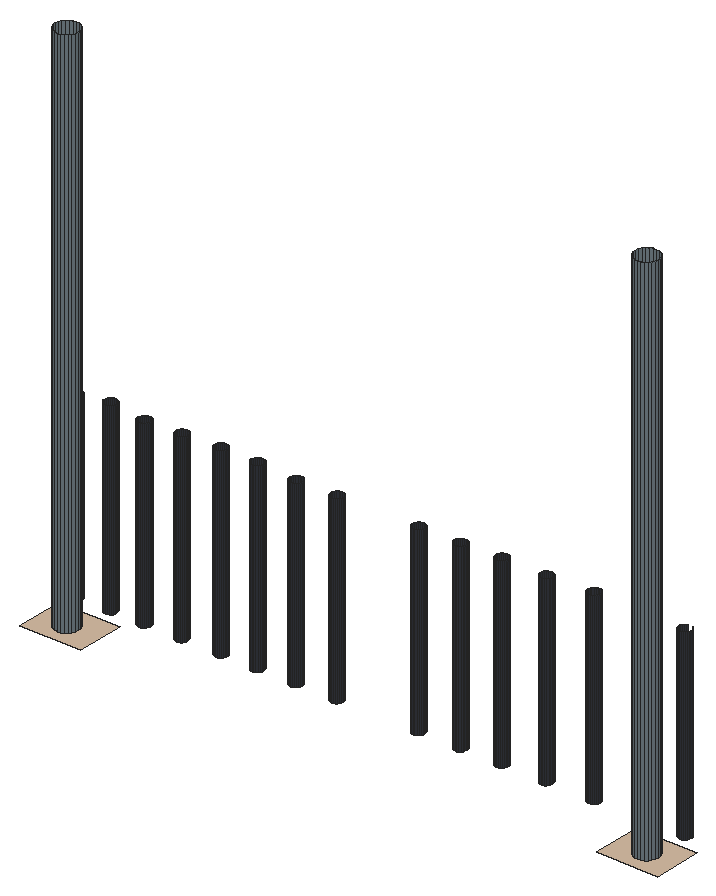
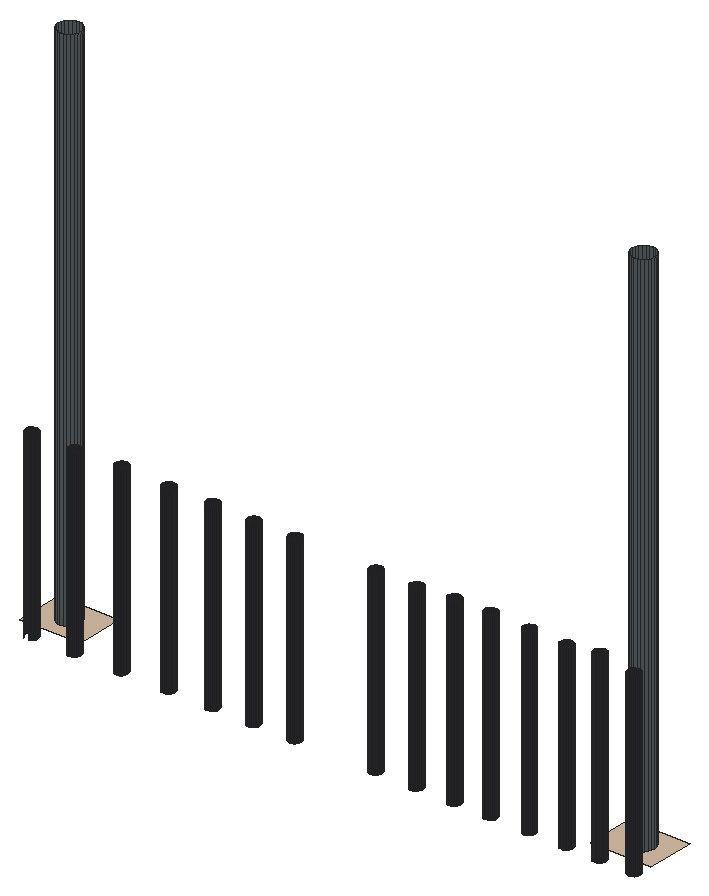
# SketchUp Ruby script. Lengths in inches.
U = 1.inch
M = Sketchup.active_model
def pt(a) = Geom::Point3d.new(a.map { |v| v * U })
def face(e, loops, mat)
  f = e.add_face(loops[0].map { |a| pt(a) })
  loops[1..].each { |l| e.add_face(l.map { |a| pt(a) }).erase! }
  f.material = f.back_material = mat if mat
  f
end
# faces: each face lists its corners as indices into pts; further lists are holes
def faces(e, pts, list, mat = nil) = list.each { |f| face(e, (f[0].is_a?(Array) ? f : [f]).map { |l| l.map { |i| pts[i] } }, mat) }
# xy, xz, yz: faces in a plane at the given z, y or x. An outline is a flat list of corners, or four numbers for a rectangle; further outlines are holes
def ring(l) = l.size == 4 ? [[l[0], l[1]], [l[2], l[1]], [l[2], l[3]], [l[0], l[3]]] : l.each_slice(2).to_a
def flat(e, list, mat, &to3) = list.each { |f| face(e, (f[0].is_a?(Array) ? f : [f]).map { |l| ring(l).map { |u, v| to3.(u, v) } }, mat) }
def xy(e, z, list, mat = nil) = flat(e, list, mat) { |x, y| [x, y, z] }
def xz(e, y, list, mat = nil) = flat(e, list, mat) { |x, z| [x, y, z] }
def yz(e, x, list, mat = nil) = flat(e, list, mat) { |y, z| [x, y, z] }
def lines(e, pts, list) = list.each { |a, b| e.add_line(pt(pts[a]), pt(pts[b])) }
# prism: a flat outline (further loops are holes) pulled along v
def prism(e, loops, v, mat = nil)
  f = face(e, loops, mat); d = Geom::Vector3d.new(v.map { |x| x * U })
  f.pushpull(f.normal.samedirection?(d) ? d.length : -d.length)
end
def box(e, o, s, mat = nil) = prism(e, [[o, [o[0] + s[0], o[1], o[2]], [o[0] + s[0], o[1] + s[1], o[2]], [o[0], o[1] + s[1], o[2]]]], [0, 0, s[2]], mat)
def at(x, y, z, deg = 0) = Geom::Transformation.translation(pt([x, y, z])) * Geom::Transformation.rotation(ORIGIN, Z_AXIS, deg.degrees)
def axes(o, x, y, z) = Geom::Transformation.new([*x, 0, *y, 0, *z, 0, *pt(o).to_a, 1])
def part(name) = M.definitions.add(name)
# library, detail: a bought-in or finely detailed component or shape, given as its bounding box
def library(name, o, s) = part(name).tap { |d| box(d.entities, o, s) }
def detail(e, o, s) = box(e.add_group.entities, o, s)
def put(e, d, t, mat = nil) = e.add_instance(d, t).tap { |i| i.material = mat if mat }
def group(e, t, mat = nil) = e.add_group.tap { |g| g.transformation = t; g.material = mat if mat }.entities
root = M.entities
M.materials.add("[Formica Laminate Dark]").color = [50, 53, 60]
M.materials.add("[Formica Laminate Light]").color = [213, 189, 164]
M.materials.add("[Formica Speckled Grey]").color = [112, 125, 132]
xy(root,372.6,[[299.55,85.05,299.16,85.1,298.8,85.25,298.49,85.49,298.25,85.8,298.1,86.17,298.05,86.55,298.1,86.94,298.25,87.3,298.49,87.61,298.8,87.85,299.16,88,299.55,88.05,299.9375,88,300.3,87.85,300.61,87.61,300.85,87.3,301,86.94,301.05,86.55,301,86.17,300.85,85.8,300.61,85.49,300.3,85.25,299.9375,85.1],[373.86,85.05,373.47,85.1,373.11,85.25,372.8,85.49,372.5625,85.8,372.41,86.17,372.36,86.55,372.41,86.94,372.5625,87.3,372.8,87.61,373.11,87.85,373.47,88,373.86,88.05,374.25,88,374.61,87.85,374.92,87.61,375.16,87.3,375.3125,86.94,375.36,86.55,375.3125,86.17,375.16,85.8,374.92,85.49,374.61,85.25,374.25,85.1]])
xy(root,372.6,[[[295.97,83.54,303.82,89.73],[299.55,85.05,299.16,85.1,298.8,85.25,298.49,85.49,298.25,85.8,298.1,86.17,298.05,86.55,298.1,86.94,298.25,87.3,298.49,87.61,298.8,87.85,299.16,88,299.55,88.05,299.9375,88,300.3,87.85,300.61,87.61,300.85,87.3,301,86.94,301.05,86.55,301,86.17,300.85,85.8,300.61,85.49,300.3,85.25,299.9375,85.1]],[[369.85,83.54,377.7,89.73],[373.86,85.05,373.47,85.1,373.11,85.25,372.8,85.49,372.5625,85.8,372.41,86.17,372.36,86.55,372.41,86.94,372.5625,87.3,372.8,87.61,373.11,87.85,373.47,88,373.86,88.05,374.25,88,374.61,87.85,374.92,87.61,375.16,87.3,375.3125,86.94,375.36,86.55,375.3125,86.17,375.16,85.8,374.92,85.49,374.61,85.25,374.25,85.1]]],"[Formica Laminate Light]")
p = [[298.8,85.25,372.6],[299.16,85.1,372.6],[299.16,85.1,441.22],[298.8,85.25,441.22],[299.55,85.05,372.6],[299.55,85.05,441.22],
  [299.9375,85.1,372.6],[299.9375,85.1,441.22],[300.3,85.25,372.6],[300.3,85.25,441.22],[373.11,85.25,372.6],[373.47,85.1,372.6],
  [373.47,85.1,441.22],[373.11,85.25,441.22],[373.86,85.05,372.6],[373.86,85.05,441.22],[374.25,85.1,372.6],[374.25,85.1,441.22],
  [374.61,85.25,372.6],[374.61,85.25,441.22],[298.49,85.49,372.6],[298.49,85.49,441.22],[300.61,85.49,372.6],[300.61,85.49,441.22],
  [372.8,85.49,372.6],[372.8,85.49,441.22],[374.92,85.49,372.6],[374.92,85.49,441.22],[298.25,85.8,372.6],[298.25,85.8,441.22],
  [300.85,85.8,372.6],[300.85,85.8,441.22],[372.5625,85.8,372.6],[372.5625,85.8,441.22],[375.16,85.8,372.6],[375.16,85.8,441.22],
  [298.1,86.17,372.6],[298.1,86.17,441.22],[301,86.17,372.6],[301,86.17,441.22],[372.41,86.17,372.6],[372.41,86.17,441.22],
  [375.3125,86.17,372.6],[375.3125,86.17,441.22],[298.05,86.55,372.6],[298.05,86.55,441.22],[301.05,86.55,372.6],[301.05,86.55,441.22],
  [372.36,86.55,372.6],[372.36,86.55,441.22],[375.36,86.55,372.6],[375.36,86.55,441.22],[298.1,86.94,372.6],[298.1,86.94,441.22],
  [301,86.94,372.6],[301,86.94,441.22],[372.41,86.94,372.6],[372.41,86.94,441.22],[375.3125,86.94,372.6],[375.3125,86.94,441.22],
  [298.25,87.3,372.6],[298.25,87.3,441.22],[300.85,87.3,372.6],[300.85,87.3,441.22],[372.5625,87.3,372.6],[372.5625,87.3,441.22],
  [375.16,87.3,372.6],[375.16,87.3,441.22],[298.49,87.61,372.6],[298.49,87.61,441.22],[300.61,87.61,372.6],[300.61,87.61,441.22],
  [372.8,87.61,372.6],[372.8,87.61,441.22],[374.92,87.61,372.6],[374.92,87.61,441.22],[298.8,87.85,372.6],[298.8,87.85,441.22],
  [300.3,87.85,372.6],[300.3,87.85,441.22],[373.11,87.85,372.6],[373.11,87.85,441.22],[374.61,87.85,372.6],[374.61,87.85,441.22],
  [299.16,88,372.6],[299.16,88,441.22],[299.9375,88,372.6],[299.9375,88,441.22],[373.47,88,372.6],[373.47,88,441.22],
  [374.25,88,372.6],[374.25,88,441.22],[299.55,88.05,372.6],[299.55,88.05,441.22],[373.86,88.05,372.6],[373.86,88.05,441.22],
  [296.23,90.98,372.6],[296.43,90.9,372.6],[296.43,90.9,395.85],[296.23,90.98,395.85],[296.64,90.87,372.6],[296.64,90.87,395.85],
  [296.85,90.9,372.6],[296.85,90.9,395.85],[297.04,90.98,372.6],[297.04,90.98,395.85],[300.67,90.98,372.6],[300.86,90.9,372.6],
  [300.86,90.9,396.5625],[300.67,90.98,396.5625],[301.07,90.87,372.6],[301.07,90.87,396.5625],[301.28,90.9,372.6],[301.28,90.9,396.5625],
  [301.48,90.98,372.6],[301.48,90.98,396.5625],[304.98,90.98,372.6],[305.18,90.9,372.6],[305.18,90.9,396.04],[304.98,90.98,396.04],
  [305.39,90.87,372.6],[305.39,90.87,396.04],[305.6,90.9,372.6],[305.6,90.9,396.04],[305.79,90.98,372.6],[305.79,90.98,396.04],
  [309.79,90.98,372.6],[309.99,90.9,372.6],[309.99,90.9,396.16],[309.79,90.98,396.16],[310.2,90.87,372.6],[310.2,90.87,396.16],
  [310.41,90.9,372.6],[310.41,90.9,396.16],[310.6,90.98,372.6],[310.6,90.98,396.16],[314.79,90.98,372.6],[314.99,90.9,372.6],
  [314.99,90.9,396.35],[314.79,90.98,396.35],[315.2,90.87,372.6],[315.2,90.87,396.35],[315.41,90.9,372.6],[315.41,90.9,396.35],
  [315.6,90.98,372.6],[315.6,90.98,396.35],[319.48,90.98,372.6],[319.68,90.9,372.6],[319.68,90.9,396.29],[319.48,90.98,396.29],
  [319.89,90.87,372.6],[319.89,90.87,396.29],[320.1,90.9,372.6],[320.1,90.9,396.29],[320.29,90.98,372.6],[320.29,90.98,396.29],
  [324.42,90.98,372.6],[324.61,90.9,372.6],[324.61,90.9,395.97],[324.42,90.98,395.97],[324.82,90.87,372.6],[324.82,90.87,395.97],
  [325.03,90.9,372.6],[325.03,90.9,395.97],[325.23,90.98,372.6],[325.23,90.98,395.97],[329.67,90.98,372.6],[329.86,90.9,372.6],
  [329.86,90.9,396.04],[329.67,90.98,396.04],[330.07,90.87,372.6],[330.07,90.87,396.04],[330.28,90.9,372.6],[330.28,90.9,396.04],
  [330.48,90.98,372.6],[330.48,90.98,396.04],[340.1,90.98,372.6],[340.3,90.9,372.6],[340.3,90.9,396.16],[340.1,90.98,396.16],
  [340.51,90.87,372.6],[340.51,90.87,396.16],[340.72,90.9,372.6],[340.72,90.9,396.16],[340.92,90.98,372.6],[340.92,90.98,396.16],
  [345.48,90.98,372.6],[345.68,90.9,372.6],[345.68,90.9,396.16],[345.48,90.98,396.16],[345.89,90.87,372.6],[345.89,90.87,396.16],
  [346.1,90.9,372.6],[346.1,90.9,396.16],[346.29,90.98,372.6],[346.29,90.98,396.16],[350.79,90.98,372.6],[350.99,90.9,372.6],
  [350.99,90.9,396.35],[350.79,90.98,396.35],[351.2,90.87,372.6],[351.2,90.87,396.35],[351.41,90.9,372.6],[351.41,90.9,396.35],
  [351.6,90.98,372.6],[351.6,90.98,396.35],[356.48,90.98,372.6],[356.68,90.9,372.6],[356.68,90.9,396.29],[356.48,90.98,396.29],
  [356.89,90.87,372.6],[356.89,90.87,396.29],[357.1,90.9,372.6],[357.1,90.9,396.29],[357.29,90.98,372.6],[357.29,90.98,396.29],
  [362.6,90.98,372.6],[362.8,90.9,372.6],[362.8,90.9,396.54],[362.6,90.98,396.54],[363.01,90.87,372.6],[363.01,90.87,396.54],
  [363.22,90.9,372.6],[363.22,90.9,396.54],[363.42,90.98,372.6],[363.42,90.98,396.54],[368.67,90.98,372.6],[368.86,90.9,372.6],
  [368.86,90.9,396.29],[368.67,90.98,396.29],[369.07,90.87,372.6],[369.07,90.87,396.29],[369.28,90.9,372.6],[369.28,90.9,396.29],
  [369.48,90.98,372.6],[369.48,90.98,396.29],[374.23,90.98,372.6],[374.43,90.9,372.6],[374.43,90.9,396.41],[374.23,90.98,396.41],
  [374.64,90.87,372.6],[374.64,90.87,396.41],[374.85,90.9,372.6],[374.85,90.9,396.41],[375.04,90.98,372.6],[375.04,90.98,396.41],
  [296.0625,91.11,372.6],[296.0625,91.11,395.85],[297.21,91.11,372.6],[297.21,91.11,395.85],[300.5,91.11,372.6],[300.61,91.03,396.5625],
  [300.5,91.11,396.5625],[300.5,91.11,395.95],[301.65,91.11,372.6],[301.65,91.11,395.95],[301.65,91.11,396.5625],[301.54,91.03,396.5625],
  [304.8125,91.11,372.6],[304.8125,91.11,396.04],[304.8125,91.11,395.95],[305.96,91.11,372.6],[305.96,91.11,395.95],[305.96,91.11,396.04],
  [309.625,91.11,372.6],[309.625,91.11,396.16],[309.625,91.11,395.95],[310.77,91.11,372.6],[310.77,91.11,395.95],[310.77,91.11,396.16],
  [314.625,91.11,372.6],[314.77,91,396.35],[314.625,91.11,396.35],[314.625,91.11,395.95],[315.77,91.11,372.6],[315.77,91.11,395.95],
  [315.77,91.11,396.35],[315.63,91,396.35],[319.3125,91.11,372.6],[319.3125,91.11,396.29],[319.3125,91.11,395.95],[320.46,91.11,372.6],
  [320.46,91.11,395.95],[320.46,91.11,396.29],[324.25,91.11,372.6],[324.25,91.11,395.97],[324.25,91.11,395.95],[325.4,91.11,372.6],
  [325.4,91.11,395.95],[325.4,91.11,395.97],[329.5,91.11,372.6],[329.5,91.11,396.04],[329.5,91.11,395.95],[330.65,91.11,372.6],
  [330.65,91.11,395.95],[330.65,91.11,396.04],[339.9375,91.11,372.6],[339.9375,91.11,396.16],[339.9375,91.11,395.95],[341.09,91.11,372.6],
  [341.09,91.11,395.95],[341.09,91.11,396.16],[345.3125,91.11,372.6],[345.3125,91.11,396.16],[345.3125,91.11,395.95],[346.46,91.11,372.6],
  [346.46,91.11,395.95],[346.46,91.11,396.16],[350.625,91.11,372.6],[350.625,91.11,396.35],[350.625,91.11,395.95],[351.77,91.11,372.6],
  [351.77,91.11,395.95],[351.77,91.11,396.35],[356.3125,91.11,372.6],[356.3125,91.11,396.29],[356.3125,91.11,395.95],[357.46,91.11,372.6],
  [357.46,91.11,395.95],[357.46,91.11,396.29],[362.4375,91.11,372.6],[362.4375,91.11,396.54],[362.4375,91.11,395.95],[363.59,91.11,372.6],
  [363.59,91.11,395.95],[363.59,91.11,396.54],[368.5,91.11,372.6],[368.5,91.11,396.29],[368.5,91.11,395.95],[369.65,91.11,372.6],
  [369.65,91.11,395.95],[369.65,91.11,396.29],[374.0625,91.11,372.6],[374.0625,91.11,396.41],[374.0625,91.11,395.95],[375.21,91.11,372.6],
  [375.21,91.11,395.95],[375.21,91.11,396.41],[295.93,91.28,372.6],[295.93,91.28,395.85],[297.34,91.28,372.6],[297.34,91.28,395.85],
  [300.37,91.28,372.6],[300.37,91.28,396.5625],[301.78,91.28,372.6],[301.78,91.28,396.5625],[304.68,91.28,372.6],[304.68,91.28,396.04],
  [306.09,91.28,372.6],[306.09,91.28,396.04],[309.49,91.28,372.6],[309.49,91.28,396.16],[310.9,91.28,372.6],[310.9,91.28,396.16],
  [314.49,91.28,372.6],[314.49,91.28,396.35],[315.9,91.28,372.6],[315.9,91.28,396.35],[319.18,91.28,372.6],[319.18,91.28,396.29],
  [320.59,91.28,372.6],[320.59,91.28,396.29],[324.12,91.28,372.6],[324.12,91.28,395.97],[325.53,91.28,372.6],[325.53,91.28,395.97],
  [329.37,91.28,372.6],[329.37,91.28,396.04],[330.78,91.28,372.6],[330.78,91.28,396.04],[339.81,91.28,372.6],[339.81,91.28,396.16],
  [341.21,91.28,372.6],[341.21,91.28,396.16],[345.18,91.28,372.6],[345.18,91.28,396.16],[346.59,91.28,372.6],[346.59,91.28,396.16],
  [350.49,91.28,372.6],[350.49,91.28,396.35],[351.9,91.28,372.6],[351.9,91.28,396.35],[356.18,91.28,372.6],[356.18,91.28,396.29],
  [357.59,91.28,372.6],[357.59,91.28,396.29],[362.31,91.28,372.6],[362.31,91.28,396.54],[363.71,91.28,372.6],[363.71,91.28,396.54],
  [368.37,91.28,372.6],[368.37,91.28,396.29],[369.78,91.28,372.6],[369.78,91.28,396.29],[373.93,91.28,372.6],[373.93,91.28,396.41],
  [375.34,91.28,372.6],[375.34,91.28,396.41],[295.85,91.47,372.6],[295.85,91.47,395.85],[297.42,91.47,372.6],[297.42,91.47,395.85],
  [300.29,91.47,372.6],[300.29,91.47,396.5625],[301.86,91.47,372.6],[301.86,91.47,396.5625],[304.6,91.47,372.6],[304.6,91.47,396.04],
  [306.17,91.47,372.6],[306.17,91.47,396.04],[309.41,91.47,372.6],[309.41,91.47,396.16],[310.98,91.47,372.6],[310.98,91.47,396.16],
  [314.41,91.47,372.6],[314.41,91.47,396.35],[315.98,91.47,372.6],[315.98,91.47,396.35],[319.1,91.47,372.6],[319.1,91.47,396.29],
  [320.67,91.47,372.6],[320.67,91.47,396.29],[324.04,91.47,372.6],[324.04,91.47,395.97],[325.61,91.47,372.6],[325.61,91.47,395.97],
  [329.29,91.47,372.6],[329.29,91.47,396.04],[330.86,91.47,372.6],[330.86,91.47,396.04],[339.73,91.47,372.6],[339.73,91.47,396.16],
  [341.3,91.47,372.6],[341.3,91.47,396.16],[345.1,91.47,372.6],[345.1,91.47,396.16],[346.67,91.47,372.6],[346.67,91.47,396.16],
  [350.41,91.47,372.6],[350.41,91.47,396.35],[351.98,91.47,372.6],[351.98,91.47,396.35],[356.1,91.47,372.6],[356.1,91.47,396.29],
  [357.67,91.47,372.6],[357.67,91.47,396.29],[362.23,91.47,372.6],[362.23,91.47,396.54],[363.8,91.47,372.6],[363.8,91.47,396.54],
  [368.29,91.47,372.6],[368.29,91.47,396.29],[369.86,91.47,372.6],[369.86,91.47,396.29],[373.85,91.47,372.6],[373.85,91.47,396.41],
  [375.42,91.47,372.6],[375.42,91.47,396.41],[295.82,91.68,372.6],[295.82,91.68,395.85],[297.45,91.68,372.6],[297.45,91.68,395.85],
  [300.26,91.68,372.6],[300.26,91.68,396.5625],[301.89,91.68,372.6],[301.89,91.68,396.5625],[304.57,91.68,372.6],[304.57,91.68,396.04],
  [306.2,91.68,372.6],[306.2,91.68,396.04],[309.39,91.68,372.6],[309.39,91.68,396.16],[311.01,91.68,372.6],[311.01,91.68,396.16],
  [314.39,91.68,372.6],[314.39,91.68,396.35],[316.01,91.68,372.6],[316.01,91.68,396.35],[319.07,91.68,372.6],[319.07,91.68,396.29],
  [320.7,91.68,372.6],[320.7,91.68,396.29],[324.01,91.68,372.6],[324.01,91.68,395.97],[325.64,91.68,372.6],[325.64,91.68,395.97],
  [329.26,91.68,372.6],[329.26,91.68,396.04],[330.89,91.68,372.6],[330.89,91.68,396.04],[339.7,91.68,372.6],[339.7,91.68,396.16],
  [341.32,91.68,372.6],[341.32,91.68,396.16],[345.07,91.68,372.6],[345.07,91.68,396.16],[346.7,91.68,372.6],[346.7,91.68,396.16],
  [350.39,91.68,372.6],[350.39,91.68,396.35],[352.01,91.68,372.6],[352.01,91.68,396.35],[356.07,91.68,372.6],[356.07,91.68,396.29],
  [357.7,91.68,372.6],[357.7,91.68,396.29],[362.2,91.68,372.6],[362.2,91.68,396.54],[363.82,91.68,372.6],[363.82,91.68,396.54],
  [368.26,91.68,372.6],[368.26,91.68,396.29],[369.89,91.68,372.6],[369.89,91.68,396.29],[373.82,91.68,372.6],[373.82,91.68,396.41],
  [375.45,91.68,372.6],[375.45,91.68,396.41],[295.85,91.89,372.6],[295.85,91.89,395.85],[297.42,91.89,372.6],[297.42,91.89,395.85],
  [300.29,91.89,372.6],[300.29,91.89,396.5625],[301.86,91.89,372.6],[301.86,91.89,396.5625],[304.6,91.89,372.6],[304.6,91.89,396.04],
  [306.17,91.89,372.6],[306.17,91.89,396.04],[309.41,91.89,372.6],[309.41,91.89,396.16],[310.98,91.89,372.6],[310.98,91.89,396.16],
  [314.41,91.89,372.6],[314.41,91.89,396.35],[315.98,91.89,372.6],[315.98,91.89,396.35],[319.1,91.89,372.6],[319.1,91.89,396.29],
  [320.67,91.89,372.6],[320.67,91.89,396.29],[324.04,91.89,372.6],[324.04,91.89,395.97],[325.61,91.89,372.6],[325.61,91.89,395.97],
  [329.29,91.89,372.6],[329.29,91.89,396.04],[330.86,91.89,372.6],[330.86,91.89,396.04],[339.73,91.89,372.6],[339.73,91.89,396.16],
  [341.3,91.89,372.6],[341.3,91.89,396.16],[345.1,91.89,372.6],[345.1,91.89,396.16],[346.67,91.89,372.6],[346.67,91.89,396.16],
  [350.41,91.89,372.6],[350.41,91.89,396.35],[351.98,91.89,372.6],[351.98,91.89,396.35],[356.1,91.89,372.6],[356.1,91.89,396.29],
  [357.67,91.89,372.6],[357.67,91.89,396.29],[362.23,91.89,372.6],[362.23,91.89,396.54],[363.8,91.89,372.6],[363.8,91.89,396.54],
  [368.29,91.89,372.6],[368.29,91.89,396.29],[369.86,91.89,372.6],[369.86,91.89,396.29],[373.85,91.89,372.6],[373.85,91.89,396.41],
  [375.42,91.89,372.6],[375.42,91.89,396.41],[295.93,92.09,372.6],[295.93,92.09,395.85],[297.34,92.09,372.6],[297.34,92.09,395.85],
  [300.37,92.09,372.6],[300.37,92.09,396.5625],[301.78,92.09,372.6],[301.78,92.09,396.5625],[304.68,92.09,372.6],[304.68,92.09,396.04],
  [306.09,92.09,372.6],[306.09,92.09,396.04],[309.49,92.09,372.6],[309.49,92.09,396.16],[310.9,92.09,372.6],[310.9,92.09,396.16],
  [314.49,92.09,372.6],[314.49,92.09,396.35],[315.9,92.09,372.6],[315.9,92.09,396.35],[319.18,92.09,372.6],[319.18,92.09,396.29],
  [320.59,92.09,372.6],[320.59,92.09,396.29],[324.12,92.09,372.6],[324.12,92.09,395.97],[325.53,92.09,372.6],[325.53,92.09,395.97],
  [329.37,92.09,372.6],[329.37,92.09,396.04],[330.78,92.09,372.6],[330.78,92.09,396.04],[339.81,92.09,372.6],[339.81,92.09,396.16],
  [341.21,92.09,372.6],[341.21,92.09,396.16],[345.18,92.09,372.6],[345.18,92.09,396.16],[346.59,92.09,372.6],[346.59,92.09,396.16],
  [350.49,92.09,372.6],[350.49,92.09,396.35],[351.9,92.09,372.6],[351.9,92.09,396.35],[356.18,92.09,372.6],[356.18,92.09,396.29],
  [357.59,92.09,372.6],[357.59,92.09,396.29],[362.31,92.09,372.6],[362.31,92.09,396.54],[363.71,92.09,372.6],[363.71,92.09,396.54],
  [368.37,92.09,372.6],[368.37,92.09,396.29],[369.78,92.09,372.6],[369.78,92.09,396.29],[373.93,92.09,372.6],[373.93,92.09,396.41],
  [375.34,92.09,372.6],[375.34,92.09,396.41],[296.0625,92.26,372.6],[296.0625,92.26,395.85],[297.21,92.26,372.6],[297.21,92.26,395.85],
  [300.5,92.26,372.6],[300.5,92.26,396.5625],[301.65,92.26,372.6],[301.65,92.26,396.5625],[304.8125,92.26,372.6],[304.8125,92.26,396.04],
  [305.96,92.26,372.6],[305.96,92.26,396.04],[309.625,92.26,372.6],[309.625,92.26,396.16],[310.77,92.26,372.6],[310.77,92.26,396.16],
  [314.625,92.26,372.6],[314.625,92.26,396.35],[315.77,92.26,372.6],[315.77,92.26,396.35],[319.3125,92.26,372.6],[319.3125,92.26,396.29],
  [320.46,92.26,372.6],[320.46,92.26,396.29],[324.25,92.26,372.6],[324.25,92.26,395.97],[325.4,92.26,372.6],[325.4,92.26,395.97],
  [329.5,92.26,372.6],[329.5,92.26,396.04],[330.65,92.26,372.6],[330.65,92.26,396.04],[339.9375,92.26,372.6],[339.9375,92.26,396.16],
  [341.09,92.26,372.6],[341.09,92.26,396.16],[345.3125,92.26,372.6],[345.3125,92.26,396.16],[346.46,92.26,372.6],[346.46,92.26,396.16],
  [350.625,92.26,372.6],[350.625,92.26,396.35],[351.77,92.26,372.6],[351.77,92.26,396.35],[356.3125,92.26,372.6],[356.3125,92.26,396.29],
  [357.46,92.26,372.6],[357.46,92.26,396.29],[362.4375,92.26,372.6],[362.4375,92.26,396.54],[363.59,92.26,372.6],[363.59,92.26,396.54],
  [368.5,92.26,372.6],[368.5,92.26,396.29],[369.65,92.26,372.6],[369.65,92.26,396.29],[374.0625,92.26,372.6],[374.0625,92.26,396.41],
  [375.21,92.26,372.6],[375.21,92.26,396.41],[296.23,92.39,372.6],[296.23,92.39,395.85],[296.23,92.39,395.78],[297.04,92.39,372.6],
  [297.04,92.39,395.78],[297.04,92.39,395.85],[300.67,92.39,372.6],[300.67,92.39,396.5625],[300.67,92.39,395.78],[301.48,92.39,372.6],
  [301.48,92.39,395.78],[301.48,92.39,396.5625],[304.98,92.39,372.6],[304.98,92.39,396.04],[304.98,92.39,395.78],[305.79,92.39,372.6],
  [305.79,92.39,395.78],[305.79,92.39,396.04],[309.79,92.39,372.6],[309.79,92.39,396.16],[309.79,92.39,395.78],[310.6,92.39,372.6],
  [310.6,92.39,395.78],[310.6,92.39,396.16],[314.79,92.39,372.6],[314.79,92.39,396.35],[314.79,92.39,395.78],[315.6,92.39,372.6],
  [315.6,92.39,395.78],[315.6,92.39,396.35],[319.48,92.39,372.6],[319.48,92.39,396.29],[319.48,92.39,395.78],[320.29,92.39,372.6],
  [320.29,92.39,395.78],[320.29,92.39,396.29],[324.42,92.39,372.6],[324.42,92.39,395.97],[324.42,92.39,395.78],[325.23,92.39,372.6],
  [325.23,92.39,395.78],[325.23,92.39,395.97],[329.67,92.39,372.6],[329.67,92.39,396.04],[329.67,92.39,395.78],[330.48,92.39,372.6],
  [330.48,92.39,395.78],[330.48,92.39,396.04],[340.1,92.39,372.6],[340.1,92.39,396.16],[340.1,92.39,395.78],[340.92,92.39,372.6],
  [340.92,92.39,395.78],[340.92,92.39,396.16],[345.48,92.39,372.6],[345.48,92.39,396.16],[345.48,92.39,395.78],[346.29,92.39,372.6],
  [346.29,92.39,395.78],[346.29,92.39,396.16],[350.79,92.39,372.6],[350.79,92.39,396.35],[350.79,92.39,395.78],[351.6,92.39,372.6],
  [351.6,92.39,395.78],[351.6,92.39,396.35],[356.48,92.39,372.6],[356.48,92.39,396.29],[356.48,92.39,395.78],[357.29,92.39,372.6],
  [357.29,92.39,395.78],[357.29,92.39,396.29],[362.6,92.39,372.6],[362.6,92.39,396.54],[362.6,92.39,395.78],[363.42,92.39,372.6],
  [363.42,92.39,395.78],[363.42,92.39,396.54],[368.67,92.39,372.6],[368.67,92.39,396.29],[368.67,92.39,395.78],[369.48,92.39,372.6],
  [369.48,92.39,395.78],[369.48,92.39,396.29],[374.23,92.39,372.6],[374.23,92.39,396.41],[374.23,92.39,395.78],[375.04,92.39,372.6],
  [375.04,92.39,395.78],[375.04,92.39,396.41],[296.43,92.47,372.6],[296.43,92.47,395.85],[296.85,92.47,372.6],[296.85,92.47,395.85],
  [300.86,92.47,372.6],[300.86,92.47,396.5625],[301.28,92.47,372.6],[301.28,92.47,396.5625],[305.18,92.47,372.6],[305.18,92.47,396.04],
  [305.6,92.47,372.6],[305.6,92.47,396.04],[309.99,92.47,372.6],[309.99,92.47,396.16],[310.41,92.47,372.6],[310.41,92.47,396.16],
  [314.99,92.47,372.6],[314.99,92.47,396.35],[315.41,92.47,372.6],[315.41,92.47,396.35],[319.68,92.47,372.6],[319.68,92.47,396.29],
  [320.1,92.47,372.6],[320.1,92.47,396.29],[324.61,92.47,372.6],[324.61,92.47,395.97],[325.03,92.47,372.6],[325.03,92.47,395.97],
  [329.86,92.47,372.6],[329.86,92.47,396.04],[330.28,92.47,372.6],[330.28,92.47,396.04],[340.3,92.47,372.6],[340.3,92.47,396.16],
  [340.72,92.47,372.6],[340.72,92.47,396.16],[345.68,92.47,372.6],[345.68,92.47,396.16],[346.1,92.47,372.6],[346.1,92.47,396.16],
  [350.99,92.47,372.6],[350.99,92.47,396.35],[351.41,92.47,372.6],[351.41,92.47,396.35],[356.68,92.47,372.6],[356.68,92.47,396.29],
  [357.1,92.47,372.6],[357.1,92.47,396.29],[362.8,92.47,372.6],[362.8,92.47,396.54],[363.22,92.47,372.6],[363.22,92.47,396.54],
  [368.86,92.47,372.6],[368.86,92.47,396.29],[369.28,92.47,372.6],[369.28,92.47,396.29],[374.43,92.47,372.6],[374.43,92.47,396.41],
  [296.64,92.5,372.6],[296.64,92.5,395.85],[301.07,92.5,372.6],[301.07,92.5,396.5625],[305.39,92.5,372.6],[305.39,92.5,396.04],
  [310.2,92.5,372.6],[310.2,92.5,396.16],[315.2,92.5,372.6],[315.2,92.5,396.35],[319.89,92.5,372.6],[319.89,92.5,396.29],
  [324.82,92.5,372.6],[324.82,92.5,395.97],[330.07,92.5,372.6],[330.07,92.5,396.04],[340.51,92.5,372.6],[340.51,92.5,396.16],
  [345.89,92.5,372.6],[345.89,92.5,396.16],[351.2,92.5,372.6],[351.2,92.5,396.35],[356.89,92.5,372.6],[356.89,92.5,396.29],
  [363.01,92.5,372.6],[363.01,92.5,396.54],[369.07,92.5,372.6],[369.07,92.5,396.29]]
faces(root,p,[[0,1,2,3],[1,4,5,2],[4,6,7,5],[6,8,9,7],[10,11,12,13],[11,14,15,12],[14,16,17,15],[16,18,19,17],
  [20,0,3,21],[8,22,23,9],[24,10,13,25],[18,26,27,19],[28,20,21,29],[22,30,31,23],[32,24,25,33],[26,34,35,27],
  [36,28,29,37],[30,38,39,31],[40,32,33,41],[34,42,43,35],[44,36,37,45],[38,46,47,39],[48,40,41,49],[42,50,51,43],
  [52,44,45,53],[46,54,55,47],[56,48,49,57],[50,58,59,51],[60,52,53,61],[54,62,63,55],[64,56,57,65],[58,66,67,59],
  [68,60,61,69],[62,70,71,63],[72,64,65,73],[66,74,75,67],[76,68,69,77],[70,78,79,71],[80,72,73,81],[74,82,83,75],
  [84,76,77,85],[78,86,87,79],[88,80,81,89],[82,90,91,83],[92,84,85,93],[86,92,93,87],[94,88,89,95],[90,94,95,91]],"[Formica Speckled Grey]")
faces(root,p,[[96,97,98,99],[97,100,101,98],[100,102,103,101],[102,104,105,103],[106,107,108,109],[107,110,111,108],[110,112,113,111],[112,114,115,113],
  [116,117,118,119],[117,120,121,118],[120,122,123,121],[122,124,125,123],[126,127,128,129],[127,130,131,128],[130,132,133,131],[132,134,135,133],
  [136,137,138,139],[137,140,141,138],[140,142,143,141],[142,144,145,143],[146,147,148,149],[147,150,151,148],[150,152,153,151],[152,154,155,153],
  [156,157,158,159],[157,160,161,158],[160,162,163,161],[162,164,165,163],[166,167,168,169],[167,170,171,168],[170,172,173,171],[172,174,175,173],
  [176,177,178,179],[177,180,181,178],[180,182,183,181],[182,184,185,183],[186,187,188,189],[187,190,191,188],[190,192,193,191],[192,194,195,193],
  [196,197,198,199],[197,200,201,198],[200,202,203,201],[202,204,205,203],[206,207,208,209],[207,210,211,208],[210,212,213,211],[212,214,215,213],
  [216,217,218,219],[217,220,221,218],[220,222,223,221],[222,224,225,223],[226,227,228,229],[227,230,231,228],[230,232,233,231],[232,234,235,233],
  [236,237,238,239],[237,240,241,238],[240,242,243,241],[242,244,245,243],[246,96,99,247],[104,248,249,105],[250,106,109,251,252,253],[114,254,255,256,257,115],
  [258,116,119,259,260],[124,261,262,263,125],[264,126,129,265,266],[134,267,268,269,135],[270,136,139,271,272,273],[144,274,275,276,277,145],[278,146,149,279,280],[154,281,282,283,155],
  [284,156,159,285,286],[164,287,288,289,165],[290,166,169,291,292],[174,293,294,295,175],[296,176,179,297,298],[184,299,300,301,185],[302,186,189,303,304],[194,305,306,307,195],
  [308,196,199,309,310],[204,311,312,313,205],[314,206,209,315,316],[214,317,318,319,215],[320,216,219,321,322],[224,323,324,325,225],[326,226,229,327,328],[234,329,330,331,235],
  [332,236,239,333,334],[244,335,336,337,245],[338,246,247,339],[248,340,341,249],[342,250,253,252,343],[254,344,345,256,255],[346,258,260,259,347],[261,348,349,263,262],
  [350,264,266,265,351],[267,352,353,269,268],[354,270,273,272,355],[274,356,357,276,275],[358,278,280,279,359],[281,360,361,283,282],[362,284,286,285,363],[287,364,365,289,288],
  [366,290,292,291,367],[293,368,369,295,294],[370,296,298,297,371],[299,372,373,301,300],[374,302,304,303,375],[305,376,377,307,306],[378,308,310,309,379],[311,380,381,313,312],
  [382,314,316,315,383],[317,384,385,319,318],[386,320,322,321,387],[323,388,389,325,324],[390,326,328,327,391],[329,392,393,331,330],[394,332,334,333,395],[335,396,397,337,336],
  [398,338,339,399],[340,400,401,341],[402,342,343,403],[344,404,405,345],[406,346,347,407],[348,408,409,349],[410,350,351,411],[352,412,413,353],
  [414,354,355,415],[356,416,417,357],[418,358,359,419],[360,420,421,361],[422,362,363,423],[364,424,425,365],[426,366,367,427],[368,428,429,369],
  [430,370,371,431],[372,432,433,373],[434,374,375,435],[376,436,437,377],[438,378,379,439],[380,440,441,381],[442,382,383,443],[384,444,445,385],
  [446,386,387,447],[388,448,449,389],[450,390,391,451],[392,452,453,393],[454,394,395,455],[396,456,457,397],[458,398,399,459],[400,460,461,401],
  [462,402,403,463],[404,464,465,405],[466,406,407,467],[408,468,469,409],[470,410,411,471],[412,472,473,413],[474,414,415,475],[416,476,477,417],
  [478,418,419,479],[420,480,481,421],[482,422,423,483],[424,484,485,425],[486,426,427,487],[428,488,489,429],[490,430,431,491],[432,492,493,433],
  [494,434,435,495],[436,496,497,437],[498,438,439,499],[440,500,501,441],[502,442,443,503],[444,504,505,445],[506,446,447,507],[448,508,509,449],
  [510,450,451,511],[452,512,513,453],[514,454,455,515],[456,516,517,457],[518,458,459,519],[460,520,521,461],[522,462,463,523],[464,524,525,465],
  [526,466,467,527],[468,528,529,469],[530,470,471,531],[472,532,533,473],[534,474,475,535],[476,536,537,477],[538,478,479,539],[480,540,541,481],
  [542,482,483,543],[484,544,545,485],[546,486,487,547],[488,548,549,489],[550,490,491,551],[492,552,553,493],[554,494,495,555],[496,556,557,497],
  [558,498,499,559],[500,560,561,501],[562,502,503,563],[504,564,565,505],[566,506,507,567],[508,568,569,509],[570,510,511,571],[512,572,573,513],
  [574,514,515,575],[516,576,577,517],[578,518,519,579],[520,580,581,521],[582,522,523,583],[524,584,585,525],[586,526,527,587],[528,588,589,529],
  [590,530,531,591],[532,592,593,533],[594,534,535,595],[536,596,597,537],[598,538,539,599],[540,600,601,541],[602,542,543,603],[544,604,605,545],
  [606,546,547,607],[548,608,609,549],[610,550,551,611],[552,612,613,553],[614,554,555,615],[556,616,617,557],[618,558,559,619],[560,620,621,561],
  [622,562,563,623],[564,624,625,565],[626,566,567,627],[568,628,629,569],[630,570,571,631],[572,632,633,573],[634,574,575,635],[576,636,637,577],
  [638,578,579,639],[580,640,641,581],[642,582,583,643],[584,644,645,585],[646,586,587,647],[588,648,649,589],[650,590,591,651],[592,652,653,593],
  [654,594,595,655],[596,656,657,597],[658,598,599,659],[600,660,661,601],[662,602,603,663],[604,664,665,605],[666,606,607,667],[608,668,669,609],
  [670,610,611,671],[612,672,673,613],[674,614,615,675],[616,676,677,617],[678,618,619,679],[620,680,681,621],[682,622,623,683],[624,684,685,625],
  [686,626,627,687],[628,688,689,629],[690,630,631,691],[632,692,693,633],[694,634,635,695],[636,696,697,637],[698,638,639,699,700],[640,701,702,703,641],
  [704,642,643,705,706],[644,707,708,709,645],[710,646,647,711,712],[648,713,714,715,649],[716,650,651,717,718],[652,719,720,721,653],[722,654,655,723,724],[656,725,726,727,657],
  [728,658,659,729,730],[660,731,732,733,661],[734,662,663,735,736],[664,737,738,739,665],[740,666,667,741,742],[668,743,744,745,669],[746,670,671,747,748],[672,749,750,751,673],
  [752,674,675,753,754],[676,755,756,757,677],[758,678,679,759,760],[680,761,762,763,681],[764,682,683,765,766],[684,767,768,769,685],[770,686,687,771,772],[688,773,774,775,689],
  [776,690,691,777,778],[692,779,780,781,693],[782,694,695,783,784],[696,785,786,787,697],[788,698,700,699,789],[701,790,791,703,702],[792,704,706,705,793],[707,794,795,709,708],
  [796,710,712,711,797],[713,798,799,715,714],[800,716,718,717,801],[719,802,803,721,720],[804,722,724,723,805],[725,806,807,727,726],[808,728,730,729,809],[731,810,811,733,732],
  [812,734,736,735,813],[737,814,815,739,738],[816,740,742,741,817],[743,818,819,745,744],[820,746,748,747,821],[749,822,823,751,750],[824,752,754,753,825],[755,826,827,757,756],
  [828,758,760,759,829],[761,830,831,763,762],[832,764,766,765,833],[767,834,835,769,768],[836,770,772,771,837],[773,838,839,775,774],[840,776,778,777,841],[779,842,843,781,780],
  [844,782,784,783,845],[846,788,789,847],[790,846,847,791],[848,792,793,849],[794,848,849,795],[850,796,797,851],[798,850,851,799],[852,800,801,853],
  [802,852,853,803],[854,804,805,855],[806,854,855,807],[856,808,809,857],[810,856,857,811],[858,812,813,859],[814,858,859,815],[860,816,817,861],
  [818,860,861,819],[862,820,821,863],[822,862,863,823],[864,824,825,865],[826,864,865,827],[866,828,829,867],[830,866,867,831],[868,832,833,869],
  [834,868,869,835],[870,836,837,871],[838,870,871,839],[872,840,841,873],[842,872,873,843]],"[Formica Laminate Dark]")
